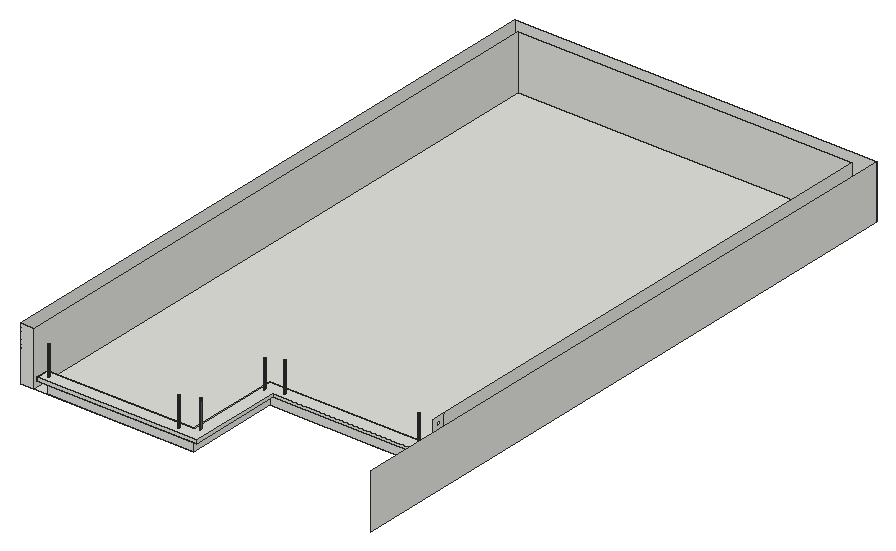
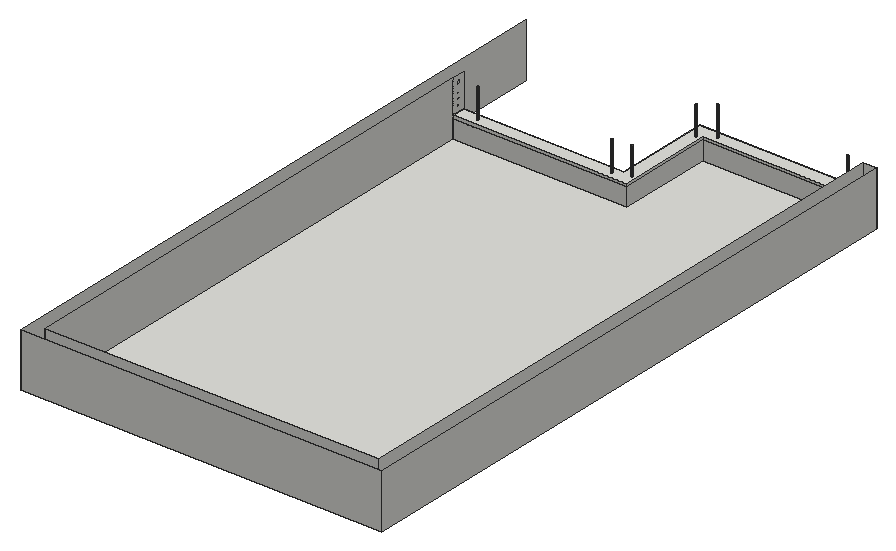
# SketchUp Ruby script. Lengths in inches.
U = 1.inch
M = Sketchup.active_model
def pt(a) = Geom::Point3d.new(a.map { |v| v * U })
def face(e, loops, mat)
  f = e.add_face(loops[0].map { |a| pt(a) })
  loops[1..].each { |l| e.add_face(l.map { |a| pt(a) }).erase! }
  f.material = f.back_material = mat if mat
  f
end
# faces: each face lists its corners as indices into pts; further lists are holes
def faces(e, pts, list, mat = nil) = list.each { |f| face(e, (f[0].is_a?(Array) ? f : [f]).map { |l| l.map { |i| pts[i] } }, mat) }
# xy, xz, yz: faces in a plane at the given z, y or x. An outline is a flat list of corners, or four numbers for a rectangle; further outlines are holes
def ring(l) = l.size == 4 ? [[l[0], l[1]], [l[2], l[1]], [l[2], l[3]], [l[0], l[3]]] : l.each_slice(2).to_a
def flat(e, list, mat, &to3) = list.each { |f| face(e, (f[0].is_a?(Array) ? f : [f]).map { |l| ring(l).map { |u, v| to3.(u, v) } }, mat) }
def xy(e, z, list, mat = nil) = flat(e, list, mat) { |x, y| [x, y, z] }
def xz(e, y, list, mat = nil) = flat(e, list, mat) { |x, z| [x, y, z] }
def yz(e, x, list, mat = nil) = flat(e, list, mat) { |y, z| [x, y, z] }
def lines(e, pts, list) = list.each { |a, b| e.add_line(pt(pts[a]), pt(pts[b])) }
# prism: a flat outline (further loops are holes) pulled along v
def prism(e, loops, v, mat = nil)
  f = face(e, loops, mat); d = Geom::Vector3d.new(v.map { |x| x * U })
  f.pushpull(f.normal.samedirection?(d) ? d.length : -d.length)
end
def box(e, o, s, mat = nil) = prism(e, [[o, [o[0] + s[0], o[1], o[2]], [o[0] + s[0], o[1] + s[1], o[2]], [o[0], o[1] + s[1], o[2]]]], [0, 0, s[2]], mat)
def at(x, y, z, deg = 0) = Geom::Transformation.translation(pt([x, y, z])) * Geom::Transformation.rotation(ORIGIN, Z_AXIS, deg.degrees)
def axes(o, x, y, z) = Geom::Transformation.new([*x, 0, *y, 0, *z, 0, *pt(o).to_a, 1])
def part(name) = M.definitions.add(name)
# library, detail: a bought-in or finely detailed component or shape, given as its bounding box
def library(name, o, s) = part(name).tap { |d| box(d.entities, o, s) }
def detail(e, o, s) = box(e.add_group.entities, o, s)
def put(e, d, t, mat = nil) = e.add_instance(d, t).tap { |i| i.material = mat if mat }
def group(e, t, mat = nil) = e.add_group.tap { |g| g.transformation = t; g.material = mat if mat }.entities
root = M.entities
M.materials.add("[Color M05]").color = [114, 114, 114]
xy(root,271.1,[[9,232.5,115.5,232.5,115.5,295.5,231,295.5,231,634.5,9,634.5]])
xy(root,283.1,[[18,223.5,18,232.5,115.5,232.5,115.5,295.5,231,295.5,231,286.5,124.5,286.5,124.5,223.5]])
xy(root,285.1,[[18,223.5,124.5,223.5,124.5,286.5,231,286.5,231,295.5,115.5,295.5,115.5,232.5,18,232.5],[22.64,227.5,22.51,227.52,22.39,227.57,22.28,227.65,22.2,227.75,22.15,227.87,22.14,228,22.15,228.13,22.2,228.25,22.28,228.35,22.39,228.43,22.51,228.48,22.64,228.5,22.77,228.48,22.89,228.43,22.99,228.35,23.07,228.25,23.12,228.13,23.14,228,23.12,227.87,23.07,227.75,22.99,227.65,22.89,227.57,22.77,227.52],[109.03,227.5,108.9,227.52,108.78,227.57,108.68,227.65,108.6,227.75,108.55,227.87,108.53,228,108.55,228.13,108.6,228.25,108.68,228.35,108.78,228.43,108.9,228.48,109.03,228.5,109.16,228.48,109.28,228.43,109.38,228.35,109.46,228.25,109.51,228.13,109.53,228,109.51,227.87,109.46,227.75,109.38,227.65,109.28,227.57,109.16,227.52],[118.73,233.14,118.6,233.15,118.48,233.2,118.375,233.28,118.3,233.38,118.24,233.5,118.23,233.63,118.24,233.76,118.29,233.88,118.37,233.99,118.47,234.07,118.59,234.12,118.72,234.14,118.85,234.12,118.97,234.07,119.08,233.99,119.16,233.89,119.21,233.77,119.23,233.64,119.21,233.51,119.16,233.39,119.08,233.28,118.98,233.2,118.86,233.15],[118.23,287.06,118.1,287.07,117.98,287.12,117.875,287.2,117.79,287.31,117.74,287.43,117.73,287.56,117.74,287.69,117.79,287.81,117.875,287.91,117.98,287.99,118.1,288.04,118.23,288.06,118.36,288.04,118.48,287.99,118.58,287.91,118.66,287.81,118.71,287.69,118.73,287.56,118.71,287.43,118.66,287.31,118.58,287.2,118.48,287.12,118.36,287.07],
  [129.01,290.5,128.88,290.52,128.76,290.57,128.66,290.65,128.58,290.75,128.53,290.87,128.51,291,128.53,291.13,128.58,291.25,128.66,291.35,128.76,291.43,128.88,291.48,129.01,291.5,129.14,291.48,129.26,291.43,129.36,291.35,129.44,291.25,129.49,291.13,129.51,291,129.49,290.87,129.44,290.75,129.36,290.65,129.26,290.57,129.14,290.52],[218.16,290.5,218.03,290.52,217.91,290.57,217.8,290.65,217.72,290.75,217.67,290.87,217.66,291,217.67,291.13,217.72,291.25,217.8,291.35,217.91,291.43,218.03,291.48,218.16,291.5,218.29,291.48,218.41,291.43,218.51,291.35,218.59,291.25,218.64,291.13,218.66,291,218.64,290.87,218.59,290.75,218.51,290.65,218.41,290.57,218.29,290.52]])
xy(root,303.6,[[118.23,287.06,118.36,287.07,118.48,287.12,118.58,287.2,118.66,287.31,118.71,287.43,118.73,287.56,118.71,287.69,118.66,287.81,118.58,287.91,118.48,287.99,118.36,288.04,118.23,288.06,118.1,288.04,117.98,287.99,117.875,287.91,117.79,287.81,117.74,287.69,117.73,287.56,117.74,287.43,117.79,287.31,117.875,287.2,117.98,287.12,118.1,287.07]])
xy(root,303.67,[[118.73,233.14,118.86,233.15,118.98,233.2,119.08,233.28,119.16,233.39,119.21,233.51,119.23,233.64,119.21,233.77,119.16,233.89,119.08,233.99,118.97,234.07,118.85,234.12,118.72,234.14,118.59,234.12,118.47,234.07,118.37,233.99,118.29,233.88,118.24,233.76,118.23,233.63,118.24,233.5,118.3,233.38,118.375,233.28,118.48,233.2,118.6,233.15]])
xy(root,304.6,[[22.64,227.5,22.77,227.52,22.89,227.57,22.99,227.65,23.07,227.75,23.12,227.87,23.14,228,23.12,228.13,23.07,228.25,22.99,228.35,22.89,228.43,22.77,228.48,22.64,228.5,22.51,228.48,22.39,228.43,22.28,228.35,22.2,228.25,22.15,228.13,22.14,228,22.15,227.87,22.2,227.75,22.28,227.65,22.39,227.57,22.51,227.52],[109.03,227.5,109.16,227.52,109.28,227.57,109.38,227.65,109.46,227.75,109.51,227.87,109.53,228,109.51,228.13,109.46,228.25,109.38,228.35,109.28,228.43,109.16,228.48,109.03,228.5,108.9,228.48,108.78,228.43,108.68,228.35,108.6,228.25,108.55,228.13,108.53,228,108.55,227.87,108.6,227.75,108.68,227.65,108.78,227.57,108.9,227.52],[129.01,290.5,129.14,290.52,129.26,290.57,129.36,290.65,129.44,290.75,129.49,290.87,129.51,291,129.49,291.13,129.44,291.25,129.36,291.35,129.26,291.43,129.14,291.48,129.01,291.5,128.88,291.48,128.76,291.43,128.66,291.35,128.58,291.25,128.53,291.13,128.51,291,128.53,290.87,128.58,290.75,128.66,290.65,128.76,290.57,128.88,290.52],[218.16,290.5,218.29,290.52,218.41,290.57,218.51,290.65,218.59,290.75,218.64,290.87,218.66,291,218.64,291.13,218.59,291.25,218.51,291.35,218.41,291.43,218.29,291.48,218.16,291.5,218.03,291.48,217.91,291.43,217.8,291.35,217.72,291.25,217.67,291.13,217.66,291,217.67,290.87,217.72,290.75,217.8,290.65,217.91,290.57,218.03,290.52]])
xz(root,223.5,[[18,283.1,124.5,285.1]])
xz(root,232.5,[[0,271.1,9,307.1],[18,271.1,115.5,283.1],[18,283.1,115.5,285.1]])
xz(root,286.5,[[124.5,283.1,231,285.1]])
xz(root,295.5,[[115.5,271.1,231,283.1],[115.5,283.1,231,285.1]])
xz(root,634.5,[[9,271.1,231,307.1]])
xz(root,643.5,[[0,271.1,240,307.1]])
yz(root,0,[[232.5,271.1,643.5,307.1]])
yz(root,9,[[232.5,271.1,634.5,307.1]])
yz(root,18,[[223.5,283.1,232.5,285.1]])
yz(root,115.5,[[232.5,271.1,295.5,283.1],[232.5,283.1,295.5,285.1]])
yz(root,124.5,[[223.5,283.1,286.5,285.1]])
yz(root,231,[[286.5,271.1,295.5,283.1],[295.5,271.1,634.5,307.1],[286.5,283.1,295.5,285.1],[[286.5,285.1,295.5,307.1],[291,301.42,291.39,301.47,291.75,301.62,292.0625,301.86,292.3,302.17,292.45,302.53,292.5,302.92,292.45,303.31,292.3,303.67,292.0625,303.98,291.75,304.22,291.39,304.37,291,304.42,290.61,304.37,290.25,304.22,289.9375,303.98,289.7,303.67,289.55,303.31,289.5,302.92,289.55,302.53,289.7,302.17,289.9375,301.86,290.25,301.62,290.61,301.47],[291,288.3125,291.26,288.34,291.5,288.44,291.71,288.6,291.87,288.8125,291.97,289.05,292,289.3125,291.97,289.57,291.87,289.8125,291.71,290.02,291.5,290.18,291.26,290.28,291,290.3125,290.74,290.28,290.5,290.18,290.29,290.02,290.13,289.8125,290.03,289.57,290,289.3125,290.03,289.05,290.13,288.8125,290.29,288.6,290.5,288.44,290.74,288.34],[291,295.92,291.26,295.95,291.5,296.05,291.71,296.21,291.87,296.42,291.97,296.66,292,296.92,291.97,297.18,291.87,297.42,291.71,297.625,291.5,297.78,291.26,297.88,291,297.92,290.74,297.88,290.5,297.78,290.29,297.625,290.13,297.42,290.03,297.18,290,296.92,290.03,296.66,290.13,296.42,290.29,296.21,290.5,296.05,290.74,295.95],[291,292.08,291.26,292.11,291.5,292.21,291.71,292.37,291.87,292.58,291.97,292.82,292,293.08,291.97,293.33,291.87,293.58,291.71,293.78,291.5,293.94,291.26,294.04,291,294.08,290.74,294.04,290.5,293.94,290.29,293.78,290.13,293.58,290.03,293.33,290,293.08,290.03,292.82,290.13,292.58,290.29,292.37,290.5,292.21,290.74,292.11]]])
yz(root,240,[[223.5,271.1,643.5,307.1]])
p = [[22.39,227.57,285.1],[22.51,227.52,285.1],[22.51,227.52,304.6],[22.39,227.57,304.6],[22.64,227.5,285.1],[22.64,227.5,304.6],
  [22.77,227.52,285.1],[22.77,227.52,304.6],[22.89,227.57,285.1],[22.89,227.57,304.6],[108.78,227.57,285.1],[108.9,227.52,285.1],
  [108.9,227.52,304.6],[108.78,227.57,304.6],[109.03,227.5,285.1],[109.03,227.5,304.6],[109.16,227.52,285.1],[109.16,227.52,304.6],
  [109.28,227.57,285.1],[109.28,227.57,304.6],[22.2,227.75,285.1],[22.28,227.65,285.1],[22.28,227.65,304.6],[22.2,227.75,304.6],
  [22.99,227.65,285.1],[22.99,227.65,304.6],[23.07,227.75,285.1],[23.07,227.75,304.6],[108.6,227.75,285.1],[108.68,227.65,285.1],
  [108.68,227.65,304.6],[108.6,227.75,304.6],[109.38,227.65,285.1],[109.38,227.65,304.6],[109.46,227.75,285.1],[109.46,227.75,304.6],
  [22.15,227.87,285.1],[22.15,227.87,304.6],[23.12,227.87,285.1],[23.12,227.87,304.6],[108.55,227.87,285.1],[108.55,227.87,304.6],
  [109.51,227.87,285.1],[109.51,227.87,304.6],[22.14,228,285.1],[22.14,228,304.6],[23.14,228,285.1],[23.14,228,304.6],
  [108.53,228,285.1],[108.53,228,304.6],[109.53,228,285.1],[109.53,228,304.6],[22.15,228.13,285.1],[22.15,228.13,304.6],
  [23.12,228.13,285.1],[23.12,228.13,304.6],[108.55,228.13,285.1],[108.55,228.13,304.6],[109.51,228.13,285.1],[109.51,228.13,304.6],
  [22.2,228.25,285.1],[22.2,228.25,304.6],[23.07,228.25,285.1],[23.07,228.25,304.6],[108.6,228.25,285.1],[108.6,228.25,304.6],
  [109.46,228.25,285.1],[109.46,228.25,304.6],[22.28,228.35,285.1],[22.28,228.35,304.6],[22.99,228.35,285.1],[22.99,228.35,304.6],
  [108.68,228.35,285.1],[108.68,228.35,304.6],[109.38,228.35,285.1],[109.38,228.35,304.6],[22.39,228.43,285.1],[22.39,228.43,304.6],
  [22.51,228.48,285.1],[22.51,228.48,304.6],[22.89,228.43,285.1],[22.77,228.48,285.1],[22.77,228.48,304.6],[22.89,228.43,304.6],
  [108.78,228.43,285.1],[108.78,228.43,304.6],[108.9,228.48,285.1],[108.9,228.48,304.6],[109.28,228.43,285.1],[109.16,228.48,285.1],
  [109.16,228.48,304.6],[109.28,228.43,304.6],[22.64,228.5,285.1],[22.64,228.5,304.6],[109.03,228.5,285.1],[109.03,228.5,304.6],
  [118.6,233.15,285.1],[118.73,233.14,285.1],[118.73,233.14,303.67],[118.6,233.15,303.67],[118.86,233.15,285.1],[118.86,233.15,303.67],
  [118.375,233.28,285.1],[118.48,233.2,285.1],[118.48,233.2,303.67],[118.375,233.28,303.67],[118.98,233.2,285.1],[118.98,233.2,303.67],
  [119.08,233.28,285.1],[119.08,233.28,303.67],[118.3,233.38,285.1],[118.3,233.38,303.67],[119.16,233.39,285.1],[119.16,233.39,303.67],
  [118.24,233.5,285.1],[118.24,233.5,303.67],[119.21,233.51,285.1],[119.21,233.51,303.67],[118.23,233.63,285.1],[118.23,233.63,303.67],
  [119.23,233.64,285.1],[119.23,233.64,303.67],[118.24,233.76,285.1],[118.24,233.76,303.67],[119.21,233.77,285.1],[119.21,233.77,303.67],
  [118.29,233.88,285.1],[118.29,233.88,303.67],[119.16,233.89,285.1],[119.16,233.89,303.67],[118.37,233.99,285.1],[118.37,233.99,303.67],
  [119.08,233.99,285.1],[119.08,233.99,303.67],[118.47,234.07,285.1],[118.47,234.07,303.67],[118.97,234.07,285.1],[118.97,234.07,303.67],
  [118.59,234.12,285.1],[118.59,234.12,303.67],[118.72,234.14,285.1],[118.72,234.14,303.67],[118.85,234.12,285.1],[118.85,234.12,303.67],
  [117.875,287.2,285.1],[117.98,287.12,285.1],[117.98,287.12,303.6],[117.875,287.2,303.6],[118.1,287.07,285.1],[118.1,287.07,303.6],
  [118.23,287.06,285.1],[118.23,287.06,303.6],[118.36,287.07,285.1],[118.36,287.07,303.6],[118.48,287.12,285.1],[118.48,287.12,303.6],
  [118.58,287.2,285.1],[118.58,287.2,303.6],[117.79,287.31,285.1],[117.79,287.31,303.6],[118.66,287.31,285.1],[118.66,287.31,303.6],
  [117.74,287.43,285.1],[117.74,287.43,303.6],[118.71,287.43,285.1],[118.71,287.43,303.6],[117.73,287.56,285.1],[117.73,287.56,303.6],
  [118.73,287.56,285.1],[118.73,287.56,303.6],[117.74,287.69,285.1],[117.74,287.69,303.6],[118.71,287.69,285.1],[118.71,287.69,303.6],
  [117.79,287.81,285.1],[117.79,287.81,303.6],[118.66,287.81,285.1],[118.66,287.81,303.6],[117.875,287.91,285.1],[117.875,287.91,303.6],
  [118.58,287.91,285.1],[118.58,287.91,303.6],[117.98,287.99,285.1],[117.98,287.99,303.6],[118.48,287.99,285.1],[118.48,287.99,303.6],
  [118.1,288.04,285.1],[118.1,288.04,303.6],[118.23,288.06,285.1],[118.23,288.06,303.6],[118.36,288.04,285.1],[118.36,288.04,303.6],
  [128.76,290.57,285.1],[128.88,290.52,285.1],[128.88,290.52,304.6],[128.76,290.57,304.6],[129.01,290.5,285.1],[129.01,290.5,304.6],
  [129.14,290.52,285.1],[129.14,290.52,304.6],[129.26,290.57,285.1],[129.26,290.57,304.6],[217.91,290.57,285.1],[218.03,290.52,285.1],
  [218.03,290.52,304.6],[217.91,290.57,304.6],[218.16,290.5,285.1],[218.16,290.5,304.6],[218.29,290.52,285.1],[218.29,290.52,304.6],
  [218.41,290.57,285.1],[218.41,290.57,304.6],[128.58,290.75,285.1],[128.66,290.65,285.1],[128.66,290.65,304.6],[128.58,290.75,304.6],
  [129.36,290.65,285.1],[129.36,290.65,304.6],[129.44,290.75,285.1],[129.44,290.75,304.6],[217.72,290.75,285.1],[217.8,290.65,285.1],
  [217.8,290.65,304.6],[217.72,290.75,304.6],[218.51,290.65,285.1],[218.51,290.65,304.6],[218.59,290.75,285.1],[218.59,290.75,304.6],
  [128.53,290.87,285.1],[128.53,290.87,304.6],[129.49,290.87,285.1],[129.49,290.87,304.6],[217.67,290.87,285.1],[217.67,290.87,304.6],
  [218.64,290.87,285.1],[218.64,290.87,304.6],[128.51,291,285.1],[128.51,291,304.6],[129.51,291,285.1],[129.51,291,304.6],
  [217.66,291,285.1],[217.66,291,304.6],[218.66,291,285.1],[218.66,291,304.6],[128.53,291.13,285.1],[128.53,291.13,304.6],
  [129.49,291.13,285.1],[129.49,291.13,304.6],[217.67,291.13,285.1],[217.67,291.13,304.6],[218.64,291.13,285.1],[218.64,291.13,304.6],
  [128.58,291.25,285.1],[128.58,291.25,304.6],[129.44,291.25,285.1],[129.44,291.25,304.6],[217.72,291.25,285.1],[217.72,291.25,304.6],
  [218.59,291.25,285.1],[218.59,291.25,304.6],[128.66,291.35,285.1],[128.66,291.35,304.6],[129.36,291.35,285.1],[129.36,291.35,304.6],
  [217.8,291.35,285.1],[217.8,291.35,304.6],[218.51,291.35,285.1],[218.51,291.35,304.6],[128.76,291.43,285.1],[128.76,291.43,304.6],
  [128.88,291.48,285.1],[128.88,291.48,304.6],[129.26,291.43,285.1],[129.14,291.48,285.1],[129.14,291.48,304.6],[129.26,291.43,304.6],
  [217.91,291.43,285.1],[217.91,291.43,304.6],[218.03,291.48,285.1],[218.03,291.48,304.6],[218.41,291.43,285.1],[218.29,291.48,285.1],
  [218.29,291.48,304.6],[218.41,291.43,304.6],[129.01,291.5,285.1],[129.01,291.5,304.6],[218.16,291.5,285.1],[218.16,291.5,304.6]]
faces(root,p,[[0,1,2,3],[1,4,5,2],[4,6,7,5],[6,8,9,7],[10,11,12,13],[11,14,15,12],[14,16,17,15],[16,18,19,17],
  [20,21,22,23],[21,0,3,22],[8,24,25,9],[24,26,27,25],[28,29,30,31],[29,10,13,30],[18,32,33,19],[32,34,35,33],
  [36,20,23,37],[26,38,39,27],[40,28,31,41],[34,42,43,35],[44,36,37,45],[38,46,47,39],[48,40,41,49],[42,50,51,43],
  [52,44,45,53],[46,54,55,47],[56,48,49,57],[50,58,59,51],[60,52,53,61],[54,62,63,55],[64,56,57,65],[58,66,67,59],
  [68,60,61,69],[62,70,71,63],[72,64,65,73],[66,74,75,67],[76,68,69,77],[78,76,77,79],[80,81,82,83],[70,80,83,71],
  [84,72,73,85],[86,84,85,87],[88,89,90,91],[74,88,91,75],[92,78,79,93],[81,92,93,82],[94,86,87,95],[89,94,95,90],
  [96,97,98,99],[97,100,101,98],[102,103,104,105],[103,96,99,104],[100,106,107,101],[106,108,109,107],[110,102,105,111],[108,112,113,109],
  [114,110,111,115],[112,116,117,113],[118,114,115,119],[116,120,121,117],[122,118,119,123],[120,124,125,121],[126,122,123,127],[124,128,129,125],
  [130,126,127,131],[128,132,133,129],[134,130,131,135],[132,136,137,133],[138,134,135,139],[140,138,139,141],[142,140,141,143],[136,142,143,137],
  [144,145,146,147],[145,148,149,146],[148,150,151,149],[150,152,153,151],[152,154,155,153],[154,156,157,155],[158,144,147,159],[156,160,161,157],
  [162,158,159,163],[160,164,165,161],[166,162,163,167],[164,168,169,165],[170,166,167,171],[168,172,173,169],[174,170,171,175],[172,176,177,173],
  [178,174,175,179],[176,180,181,177],[182,178,179,183],[180,184,185,181],[186,182,183,187],[188,186,187,189],[190,188,189,191],[184,190,191,185],
  [192,193,194,195],[193,196,197,194],[196,198,199,197],[198,200,201,199],[202,203,204,205],[203,206,207,204],[206,208,209,207],[208,210,211,209],
  [212,213,214,215],[213,192,195,214],[200,216,217,201],[216,218,219,217],[220,221,222,223],[221,202,205,222],[210,224,225,211],[224,226,227,225],
  [228,212,215,229],[218,230,231,219],[232,220,223,233],[226,234,235,227],[236,228,229,237],[230,238,239,231],[240,232,233,241],[234,242,243,235],
  [244,236,237,245],[238,246,247,239],[248,240,241,249],[242,250,251,243],[252,244,245,253],[246,254,255,247],[256,248,249,257],[250,258,259,251],
  [260,252,253,261],[254,262,263,255],[264,256,257,265],[258,266,267,259],[268,260,261,269],[270,268,269,271],[272,273,274,275],[262,272,275,263],
  [276,264,265,277],[278,276,277,279],[280,281,282,283],[266,280,283,267],[284,270,271,285],[273,284,285,274],[286,278,279,287],[281,286,287,282]],"[Color M05]")
